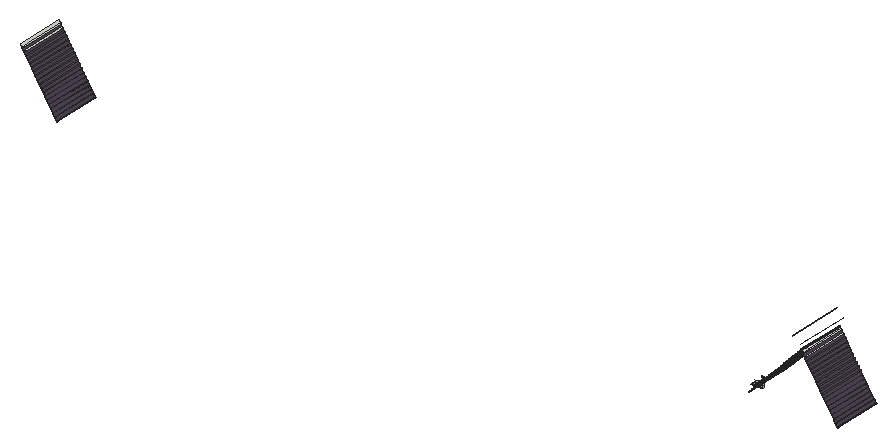
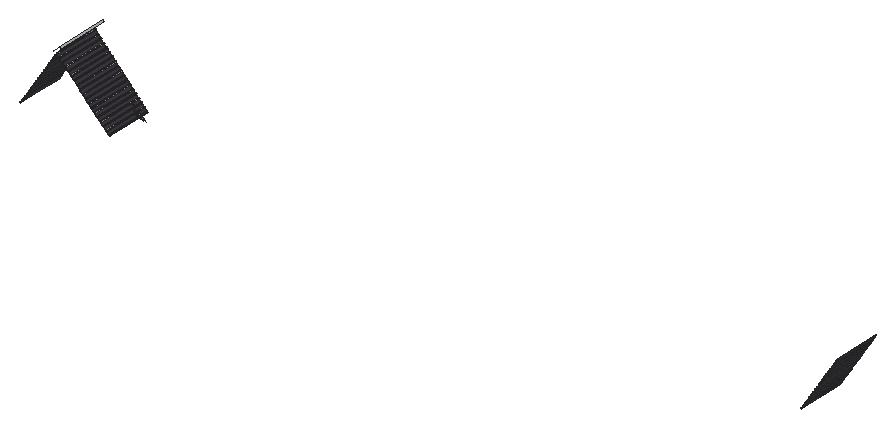
# SketchUp Ruby script. Lengths in inches.
U = 1.inch
M = Sketchup.active_model
def pt(a) = Geom::Point3d.new(a.map { |v| v * U })
def face(e, loops, mat)
  f = e.add_face(loops[0].map { |a| pt(a) })
  loops[1..].each { |l| e.add_face(l.map { |a| pt(a) }).erase! }
  f.material = f.back_material = mat if mat
  f
end
# faces: each face lists its corners as indices into pts; further lists are holes
def faces(e, pts, list, mat = nil) = list.each { |f| face(e, (f[0].is_a?(Array) ? f : [f]).map { |l| l.map { |i| pts[i] } }, mat) }
# xy, xz, yz: faces in a plane at the given z, y or x. An outline is a flat list of corners, or four numbers for a rectangle; further outlines are holes
def ring(l) = l.size == 4 ? [[l[0], l[1]], [l[2], l[1]], [l[2], l[3]], [l[0], l[3]]] : l.each_slice(2).to_a
def flat(e, list, mat, &to3) = list.each { |f| face(e, (f[0].is_a?(Array) ? f : [f]).map { |l| ring(l).map { |u, v| to3.(u, v) } }, mat) }
def xy(e, z, list, mat = nil) = flat(e, list, mat) { |x, y| [x, y, z] }
def xz(e, y, list, mat = nil) = flat(e, list, mat) { |x, z| [x, y, z] }
def yz(e, x, list, mat = nil) = flat(e, list, mat) { |y, z| [x, y, z] }
def lines(e, pts, list) = list.each { |a, b| e.add_line(pt(pts[a]), pt(pts[b])) }
# prism: a flat outline (further loops are holes) pulled along v
def prism(e, loops, v, mat = nil)
  f = face(e, loops, mat); d = Geom::Vector3d.new(v.map { |x| x * U })
  f.pushpull(f.normal.samedirection?(d) ? d.length : -d.length)
end
def box(e, o, s, mat = nil) = prism(e, [[o, [o[0] + s[0], o[1], o[2]], [o[0] + s[0], o[1] + s[1], o[2]], [o[0], o[1] + s[1], o[2]]]], [0, 0, s[2]], mat)
def at(x, y, z, deg = 0) = Geom::Transformation.translation(pt([x, y, z])) * Geom::Transformation.rotation(ORIGIN, Z_AXIS, deg.degrees)
def axes(o, x, y, z) = Geom::Transformation.new([*x, 0, *y, 0, *z, 0, *pt(o).to_a, 1])
def part(name) = M.definitions.add(name)
# library, detail: a bought-in or finely detailed component or shape, given as its bounding box
def library(name, o, s) = part(name).tap { |d| box(d.entities, o, s) }
def detail(e, o, s) = box(e.add_group.entities, o, s)
def put(e, d, t, mat = nil) = e.add_instance(d, t).tap { |i| i.material = mat if mat }
def group(e, t, mat = nil) = e.add_group.tap { |g| g.transformation = t; g.material = mat if mat }.entities
root = M.entities
M.materials.add("[Color M06]").color = [79, 71, 84]
xy(root,386.399,[[2267.279,480.141,2269.591,480.766],[2270.191,480.141,2272.503,480.766]])
xy(root,386.837,[[2267.463,480.141,2269.591,480.766],[2270.191,480.141,2272.503,480.766]])
xy(root,389.149,[[2270.191,480.141,2272.503,480.766]])
xy(root,389.587,[[2270.191,480.141,2272.503,480.766]])
xy(root,391.899,[[2272.208,480.141,2272.503,480.766]])
xy(root,397.749,[[2270.965,480.141,2273.215,480.766]])
xz(root,467.1875,[[1441.22,447.754,1441.588,447.99,1440.019,450.4375,1439.71,450.109],[2327.684,447.754,2328.052,447.99,2326.483,450.4375,2326.174,450.109],[2326.174,450.109,2326.483,450.4375,2326.115,450.201]])
xz(root,480.141,[[2261.455,385.926,2261.898,386.399,2261.455,386.399],[2264.367,386.283,2264.476,386.399,2264.367,386.399],[2260.693,386.837,2260.855,386.837,2260.855,387.008],[2261.455,386.837,2263.287,386.837,2263.767,387.346,2263.767,389.149,2262.87,389.149,2261.455,387.645],[2263.287,386.837,2263.767,386.837,2263.767,387.346],
  [2264.367,386.837,2266.679,386.837,2266.679,389.149,2265.464,389.149,2264.367,387.983],[2267.279,386.837,2267.463,386.837,2269.591,389.107,2269.591,389.149,2267.279,389.149],[2264.367,389.033,2264.476,389.149,2264.367,389.149],[2263.282,389.587,2263.767,389.587,2263.767,390.102],[2264.367,389.587,2265.876,389.587,2266.679,390.44,2266.679,391.899,2265.459,391.899,2264.367,390.739],
  [2265.876,389.587,2266.679,389.587,2266.679,390.44],[2267.279,389.587,2267.463,389.587,2269.591,391.857,2269.591,391.899,2268.053,391.899,2267.279,391.077],[2267.463,389.587,2269.591,389.587,2269.591,391.857],[2270.191,389.747,2272.208,391.899,2270.191,391.899],[2267.279,391.077,2268.053,391.899,2267.279,391.899]])
xz(root,519.6875,[[1481.241,385.328,1481.185,385.417,1481.553,385.653,1481.61,385.565],[2367.705,385.328,2367.649,385.417,2368.017,385.653,2368.074,385.565],[1479.049,388.748,1478.992,388.837,1479.36,389.073,1479.417,388.985],[2365.513,388.748,2365.456,388.837,2365.824,389.073,2365.881,388.985],[1476.856,392.168,1476.8,392.257,1477.168,392.493,1477.225,392.405],
  [2363.32,392.168,2363.264,392.257,2363.632,392.493,2363.689,392.405],[1474.664,395.588,1474.607,395.677,1474.975,395.913,1475.032,395.825],[2361.128,395.588,2361.071,395.677,2361.439,395.913,2361.496,395.825],[1472.471,399.009,1472.414,399.097,1472.783,399.333,1472.839,399.245],[2358.935,399.009,2358.878,399.097,2359.247,399.333,2359.303,399.245],
  [1470.279,402.429,1470.222,402.517,1470.59,402.753,1470.647,402.665],[2356.743,402.429,2356.686,402.517,2357.054,402.753,2357.111,402.665],[1468.086,405.849,1468.029,405.937,1468.397,406.173,1468.454,406.085],[2354.55,405.849,2354.493,405.937,2354.861,406.173,2354.918,406.085],[1465.893,409.269,1465.837,409.357,1466.205,409.593,1466.262,409.505],
  [2352.357,409.269,2352.301,409.357,2352.669,409.593,2352.726,409.505],[1463.701,412.689,1463.644,412.777,1464.012,413.013,1464.069,412.925],[2350.165,412.689,2350.108,412.777,2350.476,413.013,2350.533,412.925],[1461.508,416.109,1461.451,416.197,1461.82,416.433,1461.876,416.345],[2347.972,416.109,2347.915,416.197,2348.284,416.433,2348.34,416.345],
  [1459.316,419.529,1459.259,419.617,1459.627,419.853,1459.684,419.765],[2345.78,419.529,2345.723,419.617,2346.091,419.853,2346.148,419.765],[1457.123,422.949,1457.066,423.037,1457.434,423.273,1457.491,423.185],[2343.587,422.949,2343.53,423.037,2343.898,423.273,2343.955,423.185],[1454.93,426.369,1454.874,426.457,1455.242,426.693,1455.299,426.605],
  [2341.394,426.369,2341.338,426.457,2341.706,426.693,2341.763,426.605],[1452.738,429.789,1452.681,429.877,1453.049,430.113,1453.106,430.025],[2339.202,429.789,2339.145,429.877,2339.513,430.113,2339.57,430.025],[1450.545,433.209,1450.488,433.297,1450.857,433.533,1450.913,433.445],[2337.009,433.209,2336.952,433.297,2337.321,433.533,2337.377,433.445],
  [1448.353,436.629,1448.296,436.717,1448.664,436.953,1448.721,436.865],[2334.817,436.629,2334.76,436.717,2335.128,436.953,2335.185,436.865],[1446.16,440.049,1446.103,440.137,1446.472,440.373,1446.528,440.285],[2332.624,440.049,2332.567,440.137,2332.936,440.373,2332.992,440.285],[1443.967,443.469,1443.911,443.557,1444.279,443.793,1444.336,443.705],
  [2330.431,443.469,2330.375,443.557,2330.743,443.793,2330.8,443.705],[1441.775,446.889,1441.718,446.977,1442.086,447.213,1442.143,447.125],[2328.239,446.889,2328.182,446.977,2328.55,447.213,2328.607,447.125]])
yz(root,2269.591,[[480.141,386.837,480.766,389.107]])
yz(root,2270.191,[[480.141,386.837,480.766,389.149],[480.141,389.587,480.766,389.747]])
yz(root,2272.503,[[480.141,386.837,480.766,389.149],[480.141,389.587,480.766,391.899]])
p = [[1481.61,519.6875,385.565],[1481.61,521.5625,385.565],[1481.241,521.5625,385.328],[1481.241,519.6875,385.328],[2368.074,519.6875,385.565],[2368.074,521.5625,385.565],
  [2367.705,521.5625,385.328],[2367.705,519.6875,385.328],[1481.553,467.1875,385.653],[1481.553,519.6875,385.653],[1481.185,519.6875,385.417],[1481.185,467.1875,385.417],
  [2368.017,467.1875,385.653],[2368.017,519.6875,385.653],[2367.649,519.6875,385.417],[2367.649,467.1875,385.417],[1478.992,467.1875,388.837],[1478.992,519.6875,388.837],
  [1479.049,519.6875,388.748],[1479.049,521.5625,388.748],[1480.687,521.5625,386.194],[1480.687,467.1875,386.194],[1481.055,521.5625,386.43],[1481.055,467.1875,386.43],
  [2365.456,467.1875,388.837],[2365.456,519.6875,388.837],[2365.513,519.6875,388.748],[2365.513,521.5625,388.748],[2367.151,521.5625,386.194],[2367.151,467.1875,386.194],
  [2367.519,521.5625,386.43],[2367.519,467.1875,386.43],[2266.531,521.5625,386.746],[2266.531,467.1875,386.746],[2266.986,467.1875,386.318],[2266.986,521.5625,386.318],
  [2267.408,521.5625,387.679],[2267.408,467.1875,387.679],[2269.591,480.141,389.107],[2267.463,480.141,386.837],[2267.463,480.766,386.837],[2269.591,480.766,389.107],
  [2267.863,521.5625,387.25],[2267.863,467.1875,387.25],[2270.285,521.5625,389.822],[2270.285,467.1875,389.822],[1479.417,519.6875,388.985],[1479.417,521.5625,388.985],
  [2365.881,519.6875,388.985],[2365.881,521.5625,388.985],[1479.36,467.1875,389.073],[1479.36,519.6875,389.073],[2365.824,467.1875,389.073],[2365.824,519.6875,389.073],
  [1476.8,467.1875,392.257],[1476.8,519.6875,392.257],[1476.856,519.6875,392.168],[1476.856,521.5625,392.168],[1478.494,521.5625,389.614],[1478.494,467.1875,389.614],
  [1478.862,521.5625,389.85],[1478.862,467.1875,389.85],[2363.264,467.1875,392.257],[2363.264,519.6875,392.257],[2363.32,519.6875,392.168],[2363.32,521.5625,392.168],
  [2364.958,521.5625,389.614],[2364.958,467.1875,389.614],[2365.326,521.5625,389.85],[2365.326,467.1875,389.85],[2272.208,480.141,391.899],[2270.191,480.141,389.747],
  [2270.191,480.766,389.747],[2272.208,480.766,391.899],[2269.829,521.5625,390.251],[2269.829,467.1875,390.251],[2270.707,521.5625,391.183],[2270.707,467.1875,391.183],
  [2271.162,521.5625,390.754],[2271.162,467.1875,390.754],[2273.583,521.5625,393.327],[2273.583,467.1875,393.327],[1477.225,519.6875,392.405],[1477.225,521.5625,392.405],
  [1477.168,467.1875,392.493],[1477.168,519.6875,392.493],[2363.632,467.1875,392.493],[2363.632,519.6875,392.493],[1474.607,467.1875,395.677],[1474.607,519.6875,395.677],
  [1474.664,519.6875,395.588],[1474.664,521.5625,395.588],[1476.301,521.5625,393.034],[1476.301,467.1875,393.034],[1476.67,521.5625,393.27],[1476.67,467.1875,393.27],
  [2361.071,467.1875,395.677],[2361.071,519.6875,395.677],[2361.128,519.6875,395.588],[2361.128,521.5625,395.588],[2362.765,521.5625,393.034],[2362.765,467.1875,393.034],
  [2363.134,521.5625,393.27],[2363.134,467.1875,393.27],[2273.128,521.5625,393.755],[2273.128,467.1875,393.755],[2274.005,521.5625,394.687],[2274.005,467.1875,394.687],
  [2274.461,521.5625,394.259],[2274.461,467.1875,394.259],[2276.882,521.5625,396.831],[2276.882,467.1875,396.831],[1475.032,519.6875,395.825],[1475.032,521.5625,395.825],
  [1474.975,467.1875,395.913],[1474.975,519.6875,395.913],[2361.439,467.1875,395.913],[2361.439,519.6875,395.913],[1472.414,467.1875,399.097],[1472.414,519.6875,399.097],
  [1472.471,519.6875,399.009],[1472.471,521.5625,399.009],[1474.109,521.5625,396.454],[1474.109,467.1875,396.454],[1474.477,521.5625,396.69],[1474.477,467.1875,396.69],
  [2358.878,467.1875,399.097],[2358.878,519.6875,399.097],[2358.935,519.6875,399.009],[2358.935,521.5625,399.009],[2360.573,521.5625,396.454],[2360.573,467.1875,396.454],
  [2360.941,521.5625,396.69],[2360.941,467.1875,396.69],[2276.427,521.5625,397.259],[2276.427,467.1875,397.259],[2277.304,521.5625,398.191],[2277.304,467.1875,398.191],
  [2277.759,521.5625,397.763],[2277.759,467.1875,397.763],[2280.18,521.5625,400.335],[2280.18,467.1875,400.335],[1472.839,519.6875,399.245],[1472.839,521.5625,399.245],
  [1472.783,467.1875,399.333],[1472.783,519.6875,399.333],[2359.247,467.1875,399.333],[2359.247,519.6875,399.333],[1470.222,467.1875,402.517],[1470.222,519.6875,402.517],
  [1470.279,519.6875,402.429],[1470.279,521.5625,402.429],[1471.916,521.5625,399.874],[1471.916,467.1875,399.874],[1472.285,521.5625,400.11],[1472.285,467.1875,400.11],
  [2356.686,467.1875,402.517],[2356.686,519.6875,402.517],[2356.743,519.6875,402.429],[2356.743,521.5625,402.429],[2358.38,521.5625,399.874],[2358.38,467.1875,399.874],
  [2358.749,521.5625,400.11],[2358.749,467.1875,400.11],[2279.725,521.5625,400.763],[2279.725,467.1875,400.763],[2280.603,521.5625,401.696],[2280.603,467.1875,401.696],
  [2281.058,521.5625,401.267],[2281.058,467.1875,401.267],[2283.479,521.5625,403.839],[2283.479,467.1875,403.839],[1470.647,519.6875,402.665],[1470.647,521.5625,402.665],
  [1470.59,467.1875,402.753],[1470.59,519.6875,402.753],[2357.054,467.1875,402.753],[2357.054,519.6875,402.753],[1468.029,467.1875,405.937],[1468.029,519.6875,405.937],
  [1468.086,519.6875,405.849],[1468.086,521.5625,405.849],[1469.724,521.5625,403.294],[1469.724,467.1875,403.294],[1470.092,521.5625,403.53],[1470.092,467.1875,403.53],
  [2354.493,467.1875,405.937],[2354.493,519.6875,405.937],[2354.55,519.6875,405.849],[2354.55,521.5625,405.849],[2356.1875,521.5625,403.294],[2356.1875,467.1875,403.294],
  [2356.556,521.5625,403.53],[2356.556,467.1875,403.53],[2283.024,521.5625,404.268],[2283.024,467.1875,404.268],[2283.901,521.5625,405.2],[2283.901,467.1875,405.2],
  [2284.356,521.5625,404.771],[2284.356,467.1875,404.771],[2286.777,521.5625,407.344],[2286.777,467.1875,407.344],[1468.454,519.6875,406.085],[1468.454,521.5625,406.085],
  [1468.397,467.1875,406.173],[1468.397,519.6875,406.173],[2354.861,467.1875,406.173],[2354.861,519.6875,406.173],[1465.837,467.1875,409.357],[1465.837,519.6875,409.357],
  [1465.893,519.6875,409.269],[1465.893,521.5625,409.269],[1467.531,521.5625,406.714],[1467.531,467.1875,406.714],[1467.899,521.5625,406.95],[1467.899,467.1875,406.95],
  [2352.301,467.1875,409.357],[2352.301,519.6875,409.357],[2352.357,519.6875,409.269],[2352.357,521.5625,409.269],[2353.995,521.5625,406.714],[2353.995,467.1875,406.714],
  [2354.363,521.5625,406.95],[2354.363,467.1875,406.95],[2286.322,521.5625,407.772],[2286.322,467.1875,407.772],[2287.2,521.5625,408.704],[2287.2,467.1875,408.704],
  [2287.655,521.5625,408.276],[2287.655,467.1875,408.276],[2290.076,521.5625,410.848],[2290.076,467.1875,410.848],[1466.262,519.6875,409.505],[1466.262,521.5625,409.505],
  [1466.205,467.1875,409.593],[1466.205,519.6875,409.593],[2352.669,467.1875,409.593],[2352.669,519.6875,409.593],[1463.644,467.1875,412.777],[1463.644,519.6875,412.777],
  [1463.701,519.6875,412.689],[1463.701,521.5625,412.689],[1463.999,521.5625,412.223],[1464.151,521.5625,411.987],[1465.338,521.5625,410.134],[1465.338,467.1875,410.134],
  [1465.707,521.5625,410.37],[1465.707,467.1875,410.37],[2350.108,467.1875,412.777],[2350.108,519.6875,412.777],[2350.165,519.6875,412.689],[2350.165,521.5625,412.689],
  [2350.463,521.5625,412.223],[2350.615,521.5625,411.987],[2351.802,521.5625,410.134],[2351.802,467.1875,410.134],[2352.171,521.5625,410.37],[2352.171,467.1875,410.37],
  [2289.621,521.5625,411.276],[2289.621,467.1875,411.276],[2290.498,521.5625,412.208],[2290.498,467.1875,412.208],[2290.953,521.5625,411.78],[2290.953,467.1875,411.78],
  [2293.374,521.5625,414.352],[2293.374,467.1875,414.352],[1464.069,519.6875,412.925],[1464.069,521.5625,412.925],[2350.533,519.6875,412.925],[2350.533,521.5625,412.925],
  [1464.012,467.1875,413.013],[1464.012,519.6875,413.013],[2350.476,467.1875,413.013],[2350.476,519.6875,413.013],[1463.514,467.1875,413.79],[1463.514,521.5625,413.79],
  [2349.978,467.1875,413.79],[2349.978,521.5625,413.79],[1461.451,467.1875,416.197],[1461.451,519.6875,416.197],[1461.508,519.6875,416.109],[1461.508,521.5625,416.109],
  [1461.958,521.5625,415.407],[1463.146,521.5625,413.554],[1463.146,467.1875,413.554],[2347.915,467.1875,416.197],[2347.915,519.6875,416.197],[2347.972,519.6875,416.109],
  [2347.972,521.5625,416.109],[2348.422,521.5625,415.407],[2349.61,521.5625,413.554],[2349.61,467.1875,413.554],[2292.919,521.5625,414.78],[2292.919,467.1875,414.78],
  [2293.797,521.5625,415.713],[2293.797,467.1875,415.713],[2294.252,521.5625,415.284],[2294.252,467.1875,415.284],[2296.673,521.5625,417.856],[2296.673,467.1875,417.856],
  [1461.876,519.6875,416.345],[1461.876,521.5625,416.345],[2348.34,519.6875,416.345],[2348.34,521.5625,416.345],[1461.82,467.1875,416.433],[1461.82,519.6875,416.433],
  [2348.284,467.1875,416.433],[2348.284,519.6875,416.433],[1461.322,467.1875,417.21],[1461.322,521.5625,417.21],[2347.786,467.1875,417.21],[2347.786,521.5625,417.21],
  [1459.259,467.1875,419.617],[1459.259,519.6875,419.617],[1459.316,519.6875,419.529],[1459.316,521.5625,419.529],[1459.765,521.5625,418.827],[1460.953,521.5625,416.974],
  [1460.953,467.1875,416.974],[2345.723,467.1875,419.617],[2345.723,519.6875,419.617],[2345.78,519.6875,419.529],[2345.78,521.5625,419.529],[2346.229,521.5625,418.827],
  [2347.417,521.5625,416.974],[2347.417,467.1875,416.974],[2296.218,521.5625,418.285],[2296.218,467.1875,418.285],[2297.095,521.5625,419.217],[2297.095,467.1875,419.217],
  [2297.55,521.5625,418.788],[2297.55,467.1875,418.788],[2299.971,521.5625,421.361],[2299.971,467.1875,421.361],[1459.684,519.6875,419.765],[1459.684,521.5625,419.765],
  [2346.148,519.6875,419.765],[2346.148,521.5625,419.765],[1459.627,467.1875,419.853],[1459.627,519.6875,419.853],[2346.091,467.1875,419.853],[2346.091,519.6875,419.853],
  [1459.129,467.1875,420.63],[1459.129,521.5625,420.63],[2345.593,467.1875,420.63],[2345.593,521.5625,420.63],[1457.066,467.1875,423.037],[1457.066,519.6875,423.037],
  [1457.123,519.6875,422.949],[1457.123,521.5625,422.949],[1457.573,521.5625,422.247],[1458.761,521.5625,420.394],[1458.761,467.1875,420.394],[2343.53,467.1875,423.037],
  [2343.53,519.6875,423.037],[2343.587,519.6875,422.949],[2343.587,521.5625,422.949],[2344.037,521.5625,422.247],[2345.225,521.5625,420.394],[2345.225,467.1875,420.394],
  [2299.516,521.5625,421.789],[2299.516,467.1875,421.789],[2300.394,521.5625,422.721],[2300.394,467.1875,422.721],[2300.849,521.5625,422.293],[2300.849,467.1875,422.293],
  [2303.27,521.5625,424.865],[2303.27,467.1875,424.865],[1457.491,519.6875,423.185],[1457.491,521.5625,423.185],[2343.955,519.6875,423.185],[2343.955,521.5625,423.185],
  [1457.434,467.1875,423.273],[1457.434,519.6875,423.273],[2343.898,467.1875,423.273],[2343.898,519.6875,423.273],[1456.936,467.1875,424.05],[1456.936,521.5625,424.05],
  [2343.4,467.1875,424.05],[2343.4,521.5625,424.05],[1454.874,467.1875,426.457],[1454.874,519.6875,426.457],[1454.93,519.6875,426.369],[1454.93,521.5625,426.369],
  [1455.38,521.5625,425.667],[1456.568,521.5625,423.814],[1456.568,467.1875,423.814],[2341.338,467.1875,426.457],[2341.338,519.6875,426.457],[2341.394,519.6875,426.369],
  [2341.394,521.5625,426.369],[2341.844,521.5625,425.667],[2343.032,521.5625,423.814],[2343.032,467.1875,423.814],[2302.815,521.5625,425.293],[2302.815,467.1875,425.293],
  [2303.692,521.5625,426.225],[2303.692,467.1875,426.225],[2304.147,521.5625,425.797],[2304.147,467.1875,425.797],[2306.569,521.5625,428.369],[2306.569,467.1875,428.369],
  [1455.299,519.6875,426.605],[1455.299,521.5625,426.605],[2341.763,519.6875,426.605],[2341.763,521.5625,426.605],[1455.242,467.1875,426.693],[1455.242,519.6875,426.693],
  [2341.706,467.1875,426.693],[2341.706,519.6875,426.693],[1454.744,467.1875,427.47],[1454.744,521.5625,427.47],[2341.208,467.1875,427.47],[2341.208,521.5625,427.47],
  [1452.681,467.1875,429.877],[1452.681,519.6875,429.877],[1452.738,519.6875,429.789],[1452.738,521.5625,429.789],[1453.1875,521.5625,429.087],[1454.375,521.5625,427.234],
  [1454.375,467.1875,427.234],[2339.145,467.1875,429.877],[2339.145,519.6875,429.877],[2339.202,519.6875,429.789],[2339.202,521.5625,429.789],[2339.652,521.5625,429.087],
  [2340.839,521.5625,427.234],[2340.839,467.1875,427.234],[2306.113,521.5625,428.797],[2306.113,467.1875,428.797],[2306.991,521.5625,429.73],[2306.991,467.1875,429.73],
  [2307.446,521.5625,429.301],[2307.446,467.1875,429.301],[2309.867,521.5625,431.873],[2309.867,467.1875,431.873],[1453.106,519.6875,430.025],[1453.106,521.5625,430.025],
  [2339.57,519.6875,430.025],[2339.57,521.5625,430.025],[1453.049,467.1875,430.113],[1453.049,519.6875,430.113],[2339.513,467.1875,430.113],[2339.513,519.6875,430.113],
  [1452.551,467.1875,430.89],[1452.551,521.5625,430.89],[2339.015,467.1875,430.89],[2339.015,521.5625,430.89],[1450.488,467.1875,433.297],[1450.488,519.6875,433.297],
  [1450.545,519.6875,433.209],[1450.545,521.5625,433.209],[1450.995,521.5625,432.507],[1452.183,521.5625,430.654],[1452.183,467.1875,430.654],[2336.952,467.1875,433.297],
  [2336.952,519.6875,433.297],[2337.009,519.6875,433.209],[2337.009,521.5625,433.209],[2337.459,521.5625,432.507],[2338.647,521.5625,430.654],[2338.647,467.1875,430.654],
  [2309.412,521.5625,432.302],[2309.412,467.1875,432.302],[2310.289,521.5625,433.234],[2310.289,467.1875,433.234],[2310.745,521.5625,432.805],[2310.745,467.1875,432.805],
  [2313.166,521.5625,435.378],[2313.166,467.1875,435.378],[1450.913,519.6875,433.445],[1450.913,521.5625,433.445],[2337.377,519.6875,433.445],[2337.377,521.5625,433.445],
  [1450.857,467.1875,433.533],[1450.857,519.6875,433.533],[2337.321,467.1875,433.533],[2337.321,519.6875,433.533],[1450.359,467.1875,434.31],[1450.359,521.5625,434.31],
  [2336.823,467.1875,434.31],[2336.823,521.5625,434.31],[1448.296,467.1875,436.717],[1448.296,519.6875,436.717],[1448.353,519.6875,436.629],[1448.353,521.5625,436.629],
  [1448.802,521.5625,435.927],[1449.99,521.5625,434.074],[1449.99,467.1875,434.074],[2334.76,467.1875,436.717],[2334.76,519.6875,436.717],[2334.817,519.6875,436.629],
  [2334.817,521.5625,436.629],[2335.266,521.5625,435.927],[2336.454,521.5625,434.074],[2336.454,467.1875,434.074],[2312.711,521.5625,435.806],[2312.711,467.1875,435.806],
  [2313.588,521.5625,436.738],[2313.588,467.1875,436.738],[2314.043,521.5625,436.31],[2314.043,467.1875,436.31],[2316.464,521.5625,438.882],[2316.464,467.1875,438.882],
  [1448.721,519.6875,436.865],[1448.721,521.5625,436.865],[2335.185,519.6875,436.865],[2335.185,521.5625,436.865],[1448.664,467.1875,436.953],[1448.664,519.6875,436.953],
  [2335.128,467.1875,436.953],[2335.128,519.6875,436.953],[1448.166,467.1875,437.73],[1448.166,521.5625,437.73],[2334.63,467.1875,437.73],[2334.63,521.5625,437.73],
  [1446.103,467.1875,440.137],[1446.103,519.6875,440.137],[1446.16,519.6875,440.049],[1446.16,521.5625,440.049],[1446.61,521.5625,439.347],[1447.798,521.5625,437.494],
  [1447.798,467.1875,437.494],[2332.567,467.1875,440.137],[2332.567,519.6875,440.137],[2332.624,519.6875,440.049],[2332.624,521.5625,440.049],[2333.074,521.5625,439.347],
  [2334.262,521.5625,437.494],[2334.262,467.1875,437.494],[2316.009,521.5625,439.31],[2316.009,467.1875,439.31],[2316.887,521.5625,440.242],[2316.887,467.1875,440.242],
  [2317.342,521.5625,439.814],[2317.342,467.1875,439.814],[2319.763,521.5625,442.386],[2319.763,467.1875,442.386],[1446.528,519.6875,440.285],[1446.528,521.5625,440.285],
  [2332.992,519.6875,440.285],[2332.992,521.5625,440.285],[1446.472,467.1875,440.373],[1446.472,519.6875,440.373],[2332.936,467.1875,440.373],[2332.936,519.6875,440.373],
  [1445.973,467.1875,441.15],[1445.973,521.5625,441.15],[2332.4375,467.1875,441.15],[2332.4375,521.5625,441.15],[1443.911,467.1875,443.557],[1443.911,519.6875,443.557],
  [1443.967,519.6875,443.469],[1443.967,521.5625,443.469],[1444.417,521.5625,442.767],[1445.605,521.5625,440.914],[1445.605,467.1875,440.914],[2330.375,467.1875,443.557],
  [2330.375,519.6875,443.557],[2330.431,519.6875,443.469],[2330.431,521.5625,443.469],[2330.881,521.5625,442.767],[2332.069,521.5625,440.914],[2332.069,467.1875,440.914],
  [2319.308,521.5625,442.814],[2319.308,467.1875,442.814],[2320.185,521.5625,443.747],[2320.185,467.1875,443.747],[2320.64,521.5625,443.318],[2320.64,467.1875,443.318],
  [2323.061,521.5625,445.89],[2323.061,467.1875,445.89],[1444.336,519.6875,443.705],[1444.336,521.5625,443.705],[2330.8,519.6875,443.705],[2330.8,521.5625,443.705],
  [1444.279,467.1875,443.793],[1444.279,519.6875,443.793],[2330.743,467.1875,443.793],[2330.743,519.6875,443.793],[1443.781,467.1875,444.57],[1443.781,521.5625,444.57],
  [2330.245,467.1875,444.57],[2330.245,521.5625,444.57],[1441.718,467.1875,446.977],[1441.718,519.6875,446.977],[1441.775,519.6875,446.889],[1441.775,521.5625,446.889],
  [1442.225,521.5625,446.187],[1443.412,521.5625,444.334],[1443.412,467.1875,444.334],[2328.182,467.1875,446.977],[2328.182,519.6875,446.977],[2328.239,519.6875,446.889],
  [2328.239,521.5625,446.889],[2328.689,521.5625,446.187],[2329.876,521.5625,444.334],[2329.876,467.1875,444.334],[2322.606,521.5625,446.319],[2322.606,467.1875,446.319],
  [2323.484,521.5625,447.251],[2323.484,467.1875,447.251],[2323.939,521.5625,446.822],[2323.939,467.1875,446.822],[2326.36,521.5625,449.395],[2326.36,467.1875,449.395],
  [1442.143,519.6875,447.125],[1442.143,521.5625,447.125],[2328.607,519.6875,447.125],[2328.607,521.5625,447.125],[1442.086,467.1875,447.213],[1442.086,519.6875,447.213],
  [2328.55,467.1875,447.213],[2328.55,519.6875,447.213],[1441.588,467.1875,447.99],[1441.588,521.5625,447.99],[2328.052,467.1875,447.99],[2328.052,521.5625,447.99],
  [1440.032,521.5625,449.607],[1441.22,521.5625,447.754],[1441.22,467.1875,447.754],[1439.71,467.1875,450.109],[1439.651,467.1875,450.201],[1439.651,521.5625,450.201],
  [1439.71,521.5625,450.109],[2326.496,521.5625,449.607],[2327.684,521.5625,447.754],[2327.684,467.1875,447.754],[2326.174,467.1875,450.109],[2326.115,467.1875,450.201],
  [2326.115,521.5625,450.201],[2326.174,521.5625,450.109],[1440.4,521.5625,449.843],[1440.019,521.5625,450.4375],[1440.019,467.1875,450.4375],[2326.864,521.5625,449.843],
  [2326.483,521.5625,450.4375],[2326.483,467.1875,450.4375],[2325.905,521.5625,449.823],[2325.905,467.1875,449.823],[2326.414,521.5625,450.545],[2326.358,467.1875,450.633],
  [2326.358,519.6875,450.633],[2326.414,519.6875,450.545],[2316.577,528.483,461.307],[2316.577,467.1875,461.307],[2317.905,467.1875,462.718],[2317.905,528.483,462.718],
  [2261.455,480.141,384.89],[2261.455,480.141,385.926],[2259.321,480.141,386.399],[2260.282,480.141,386.399],[2264.476,480.141,389.149],[2265.464,480.141,389.149],
  [2261.898,480.141,386.399],[2262.876,480.141,386.399],[2258.543,480.141,385.569],[2260.855,480.141,388.036],[2260.855,480.141,387.008],[2261.898,480.141,389.149],
  [2262.87,480.141,389.149],[2261.455,480.141,387.645],[2261.455,480.141,388.676],[2260.693,480.141,386.837],[2259.731,480.141,386.837],[2264.367,480.141,387.983],
  [2263.767,480.141,387.346],[2263.287,480.141,386.837],[2264.367,480.141,389.033],[2262.87,480.141,391.899],[2262.876,480.141,391.899],[2267.279,480.141,391.077],
  [2266.679,480.141,390.44],[2265.876,480.141,389.587],[2263.282,480.141,389.587],[2262.308,480.141,389.587],[2271.781,480.141,395.86],[2268.053,480.141,391.899],
  [2272.639,480.141,395.86],[2325.442,528.483,455.623],[2325.442,467.1875,455.623]]
faces(root,p,[[0,1,2,3],[4,5,6,7],[8,9,10,11],[12,13,14,15],[22,23,21,20],[30,31,29,28],[32,33,34,35],[38,39,40,41],
  [46,47,19,18],[48,49,27,26],[50,51,17,16],[52,53,25,24],[60,61,59,58],[68,69,67,66],[70,71,72,73],[74,75,45,44],
  [77,76,78,79],[82,83,57,56],[84,85,55,54],[86,87,63,62],[94,95,93,92],[102,103,101,100],[104,105,81,80],[107,106,108,109],
  [112,113,91,90],[114,115,89,88],[116,117,97,96],[124,125,123,122],[132,133,131,130],[134,135,111,110],[137,136,138,139],[142,143,121,120],
  [144,145,119,118],[146,147,127,126],[154,155,153,152],[162,163,161,160],[164,165,141,140],[172,173,151,150],[174,175,149,148],[176,177,157,156],
  [184,185,183,182],[192,193,191,190],[194,195,171,170],[202,203,181,180],[204,205,179,178],[206,207,187,186],[214,215,213,212],[222,223,221,220],
  [224,225,201,200],[232,233,211,210],[234,235,209,208],[236,237,217,216],[246,247,245,244],[256,257,255,254],[258,259,231,230],[266,267,241,240],
  [268,269,251,250],[270,271,239,238],[272,273,249,248],[275,274,284,283],[277,276,291,290],[292,293,265,264],[300,301,281,280],[302,303,288,287],
  [304,305,279,278],[306,307,286,285],[309,308,318,317],[311,310,325,324],[326,327,299,298],[334,335,315,314],[336,337,322,321],[338,339,313,312],
  [340,341,320,319],[343,342,352,351],[345,344,359,358],[360,361,333,332],[368,369,349,348],[370,371,356,355],[372,373,347,346],[374,375,354,353],
  [377,376,386,385],[379,378,393,392],[394,395,367,366],[402,403,383,382],[404,405,390,389],[406,407,381,380],[408,409,388,387],[411,410,420,419],
  [413,412,427,426],[428,429,401,400],[431,430,432,433],[436,437,417,416],[438,439,424,423],[440,441,415,414],[442,443,422,421],[445,444,454,453],
  [447,446,461,460],[462,463,435,434],[465,464,466,467],[470,471,451,450],[472,473,458,457],[474,475,449,448],[476,477,456,455],[479,478,488,487],
  [481,480,495,494],[496,497,469,468],[499,498,500,501],[504,505,485,484],[506,507,492,491],[508,509,483,482],[510,511,490,489],[513,512,522,521],
  [515,514,529,528],[530,531,503,502],[533,532,534,535],[538,539,519,518],[540,541,526,525],[542,543,517,516],[544,545,524,523],[564,565,537,536],
  [567,566,568,569],[572,573,553,552],[574,575,560,559],[576,577,551,550],[578,579,558,557],[576,580,581,573,572,577],[578,582,583,575,574,579],[598,599,571,570],
  [601,600,602,603],[606,607,587,586],[608,609,594,593],[610,611,585,584],[612,613,592,591],[610,614,615,607,606,611],[612,616,617,609,608,613],[615,632,633,634,614],
  [617,635,636,637,616],[638,639,605,604],[628,639,638,631,636,637],[637,636,630,629],[640,636,637,641,642,643],[644,645,646,647]])
faces(root,p,[[16,17,18,19,20,21],[24,25,26,27,28,29],[32,36,37,33],[37,36,42,43],[42,44,45,43],[54,55,56,57,58,59],[62,63,64,65,66,67],[74,76,77,75],
  [78,80,81,79],[88,89,90,91,92,93],[96,97,98,99,100,101],[104,106,107,105],[108,110,111,109],[118,119,120,121,122,123],[126,127,128,129,130,131],[134,136,137,135],
  [138,140,141,139],[148,149,150,151,152,153],[156,157,158,159,160,161],[164,166,167,165],[167,166,168,169],[168,170,171,169],[178,179,180,181,182,183],[186,187,188,189,190,191],
  [194,196,197,195],[197,196,198,199],[198,200,201,199],[208,209,210,211,212,213],[216,217,218,219,220,221],[224,226,227,225],[227,226,228,229],[228,230,231,229],
  [238,239,240,241,242,243,244,245],[248,249,250,251,252,253,254,255],[258,260,261,259],[261,260,262,263],[262,264,265,263],[270,274,275,267,266,271],[272,276,277,269,268,273],[278,279,280,281,282,283,284],
  [285,286,287,288,289,290,291],[292,294,295,293],[295,294,296,297],[296,298,299,297],[304,308,309,301,300,305],[306,310,311,303,302,307],[312,313,314,315,316,317,318],[319,320,321,322,323,324,325],
  [326,328,329,327],[329,328,330,331],[330,332,333,331],[338,342,343,335,334,339],[340,344,345,337,336,341],[346,347,348,349,350,351,352],[353,354,355,356,357,358,359],[360,362,363,361],
  [363,362,364,365],[364,366,367,365],[372,376,377,369,368,373],[374,378,379,371,370,375],[380,381,382,383,384,385,386],[387,388,389,390,391,392,393],[394,396,397,395],[397,396,398,399],
  [398,400,401,399],[406,410,411,403,402,407],[408,412,413,405,404,409],[414,415,416,417,418,419,420],[421,422,423,424,425,426,427],[428,430,431,429],[432,434,435,433],[440,444,445,437,436,441],
  [442,446,447,439,438,443],[448,449,450,451,452,453,454],[455,456,457,458,459,460,461],[462,464,465,463],[466,468,469,467],[474,478,479,471,470,475],[476,480,481,473,472,477],[482,483,484,485,486,487,488],
  [489,490,491,492,493,494,495],[496,498,499,497],[500,502,503,501],[508,512,513,505,504,509],[510,514,515,507,506,511],[516,517,518,519,520,521,522],[523,524,525,526,527,528,529],[530,532,533,531],
  [534,536,537,535],[542,546,547,539,538,543],[544,548,549,541,540,545],[550,551,552,553,554,555,556],[547,546,556,555],[557,558,559,560,561,562,563],[549,548,563,562],[564,566,567,565],
  [568,570,571,569],[584,585,586,587,588,589,590],[581,580,590,589],[591,592,593,594,595,596,597],[583,582,597,596],[598,600,601,599],[602,604,605,603],[618,619,620,621,622,623,624],
  [615,614,620,619],[625,626,627,628,629,630,631],[617,616,627,626]],"[Color M06]")
lines(root,p,[[648,649],[650,651],[652,653],[654,655],[650,656],[657,658],[659,660],[661,662],[663,664],[665,666],[667,655],[665,668],
  [669,670],[671,672],[673,653],[674,675],[676,677],[678,676],[679,680]])
